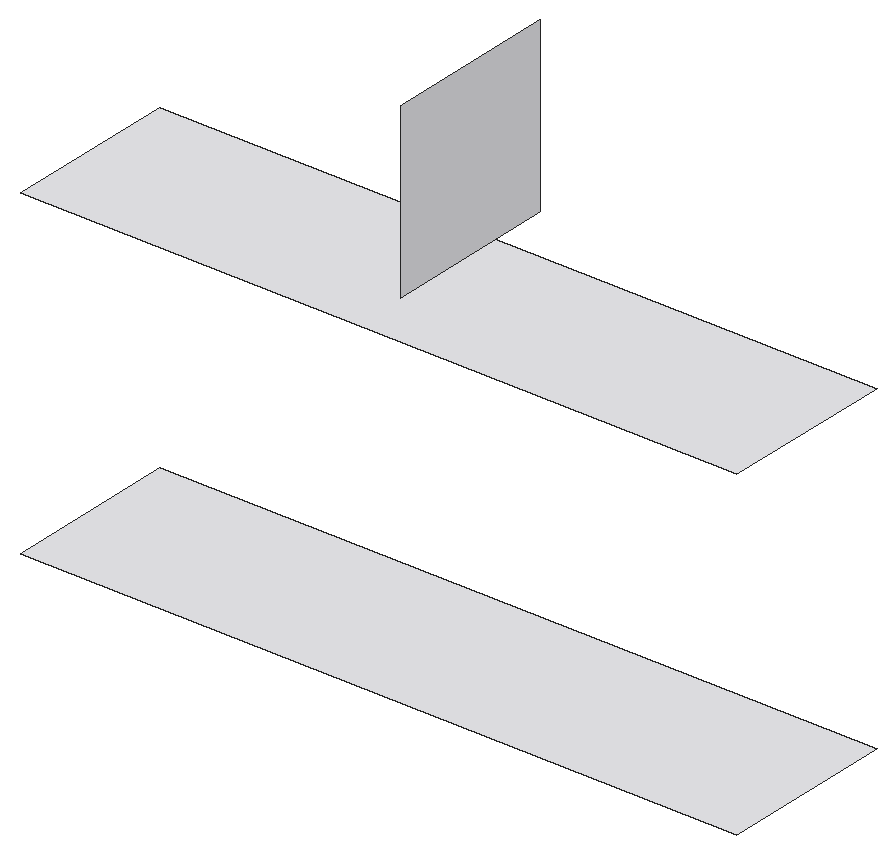
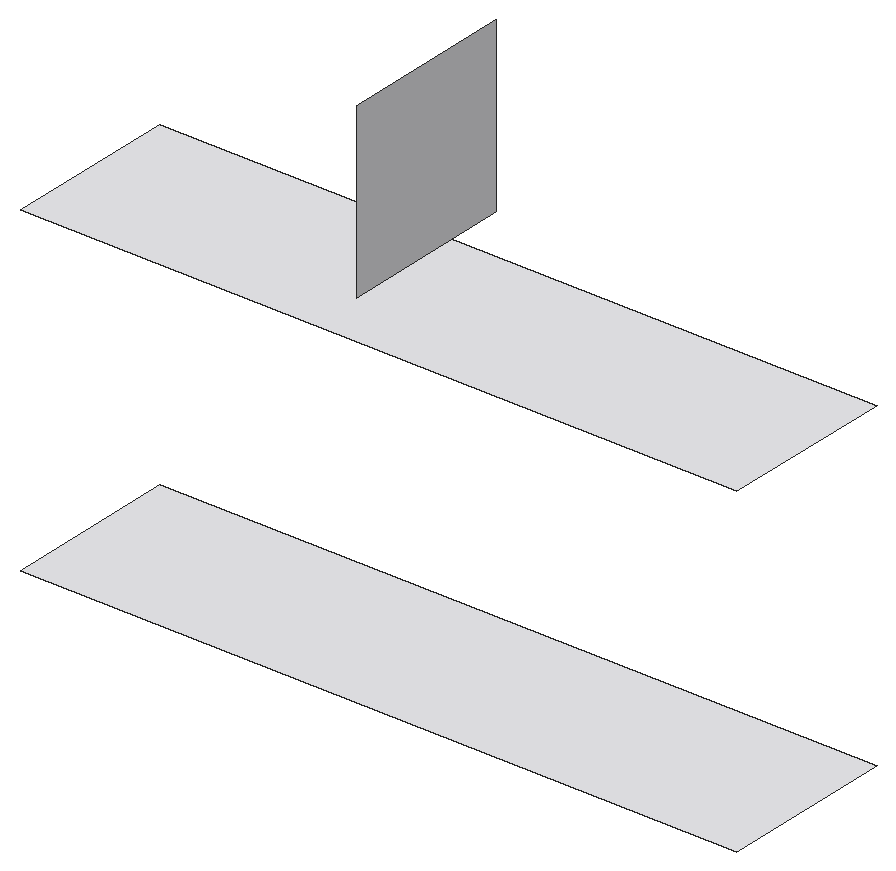
# SketchUp Ruby script. Lengths in inches.
U = 1.inch
M = Sketchup.active_model
def pt(a) = Geom::Point3d.new(a.map { |v| v * U })
def face(e, loops, mat)
  f = e.add_face(loops[0].map { |a| pt(a) })
  loops[1..].each { |l| e.add_face(l.map { |a| pt(a) }).erase! }
  f.material = f.back_material = mat if mat
  f
end
# faces: each face lists its corners as indices into pts; further lists are holes
def faces(e, pts, list, mat = nil) = list.each { |f| face(e, (f[0].is_a?(Array) ? f : [f]).map { |l| l.map { |i| pts[i] } }, mat) }
# xy, xz, yz: faces in a plane at the given z, y or x. An outline is a flat list of corners, or four numbers for a rectangle; further outlines are holes
def ring(l) = l.size == 4 ? [[l[0], l[1]], [l[2], l[1]], [l[2], l[3]], [l[0], l[3]]] : l.each_slice(2).to_a
def flat(e, list, mat, &to3) = list.each { |f| face(e, (f[0].is_a?(Array) ? f : [f]).map { |l| ring(l).map { |u, v| to3.(u, v) } }, mat) }
def xy(e, z, list, mat = nil) = flat(e, list, mat) { |x, y| [x, y, z] }
def xz(e, y, list, mat = nil) = flat(e, list, mat) { |x, z| [x, y, z] }
def yz(e, x, list, mat = nil) = flat(e, list, mat) { |y, z| [x, y, z] }
def lines(e, pts, list) = list.each { |a, b| e.add_line(pt(pts[a]), pt(pts[b])) }
# prism: a flat outline (further loops are holes) pulled along v
def prism(e, loops, v, mat = nil)
  f = face(e, loops, mat); d = Geom::Vector3d.new(v.map { |x| x * U })
  f.pushpull(f.normal.samedirection?(d) ? d.length : -d.length)
end
def box(e, o, s, mat = nil) = prism(e, [[o, [o[0] + s[0], o[1], o[2]], [o[0] + s[0], o[1] + s[1], o[2]], [o[0], o[1] + s[1], o[2]]]], [0, 0, s[2]], mat)
def at(x, y, z, deg = 0) = Geom::Transformation.translation(pt([x, y, z])) * Geom::Transformation.rotation(ORIGIN, Z_AXIS, deg.degrees)
def axes(o, x, y, z) = Geom::Transformation.new([*x, 0, *y, 0, *z, 0, *pt(o).to_a, 1])
def part(name) = M.definitions.add(name)
# library, detail: a bought-in or finely detailed component or shape, given as its bounding box
def library(name, o, s) = part(name).tap { |d| box(d.entities, o, s) }
def detail(e, o, s) = box(e.add_group.entities, o, s)
def put(e, d, t, mat = nil) = e.add_instance(d, t).tap { |i| i.material = mat if mat }
def group(e, t, mat = nil) = e.add_group.tap { |g| g.transformation = t; g.material = mat if mat }.entities
root = M.entities
M.materials.add("[Blinds Vertical Pattern]1").color = [239, 239, 242]
xy(root,7.1,[[254.71,96.24,315.3,111]],"[Blinds Vertical Pattern]1")
xy(root,34.41,[[254.71,96.24,315.3,111]],"[Blinds Vertical Pattern]1")
yz(root,286.85,[[96.24,37.78,111,52.34]],"[Blinds Vertical Pattern]1")
